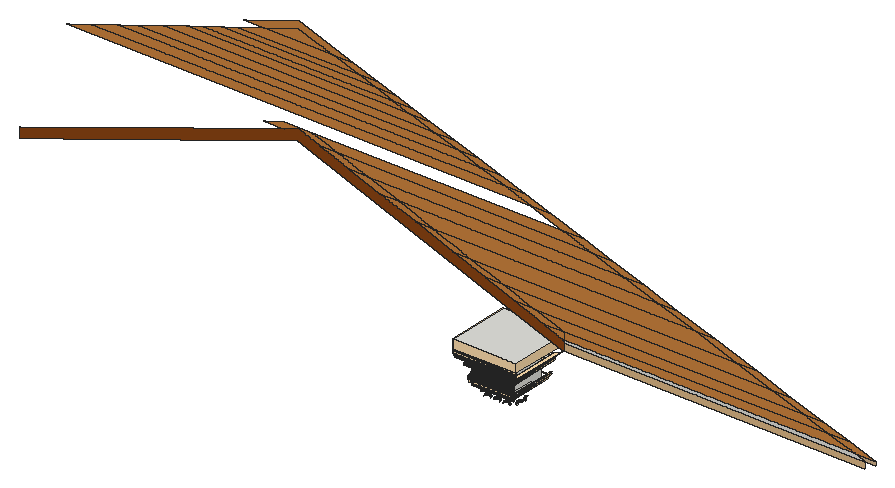
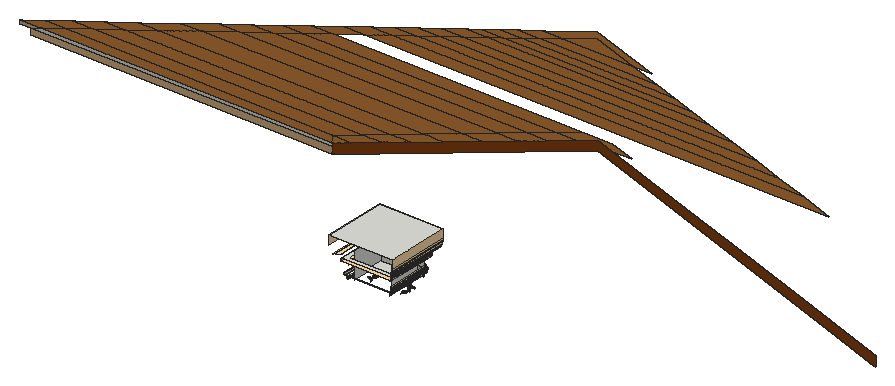
# SketchUp Ruby script. Lengths in inches.
U = 1.inch
M = Sketchup.active_model
def pt(a) = Geom::Point3d.new(a.map { |v| v * U })
def face(e, loops, mat)
  f = e.add_face(loops[0].map { |a| pt(a) })
  loops[1..].each { |l| e.add_face(l.map { |a| pt(a) }).erase! }
  f.material = f.back_material = mat if mat
  f
end
# faces: each face lists its corners as indices into pts; further lists are holes
def faces(e, pts, list, mat = nil) = list.each { |f| face(e, (f[0].is_a?(Array) ? f : [f]).map { |l| l.map { |i| pts[i] } }, mat) }
# xy, xz, yz: faces in a plane at the given z, y or x. An outline is a flat list of corners, or four numbers for a rectangle; further outlines are holes
def ring(l) = l.size == 4 ? [[l[0], l[1]], [l[2], l[1]], [l[2], l[3]], [l[0], l[3]]] : l.each_slice(2).to_a
def flat(e, list, mat, &to3) = list.each { |f| face(e, (f[0].is_a?(Array) ? f : [f]).map { |l| ring(l).map { |u, v| to3.(u, v) } }, mat) }
def xy(e, z, list, mat = nil) = flat(e, list, mat) { |x, y| [x, y, z] }
def xz(e, y, list, mat = nil) = flat(e, list, mat) { |x, z| [x, y, z] }
def yz(e, x, list, mat = nil) = flat(e, list, mat) { |y, z| [x, y, z] }
def lines(e, pts, list) = list.each { |a, b| e.add_line(pt(pts[a]), pt(pts[b])) }
# prism: a flat outline (further loops are holes) pulled along v
def prism(e, loops, v, mat = nil)
  f = face(e, loops, mat); d = Geom::Vector3d.new(v.map { |x| x * U })
  f.pushpull(f.normal.samedirection?(d) ? d.length : -d.length)
end
def box(e, o, s, mat = nil) = prism(e, [[o, [o[0] + s[0], o[1], o[2]], [o[0] + s[0], o[1] + s[1], o[2]], [o[0], o[1] + s[1], o[2]]]], [0, 0, s[2]], mat)
def at(x, y, z, deg = 0) = Geom::Transformation.translation(pt([x, y, z])) * Geom::Transformation.rotation(ORIGIN, Z_AXIS, deg.degrees)
def axes(o, x, y, z) = Geom::Transformation.new([*x, 0, *y, 0, *z, 0, *pt(o).to_a, 1])
def part(name) = M.definitions.add(name)
# library, detail: a bought-in or finely detailed component or shape, given as its bounding box
def library(name, o, s) = part(name).tap { |d| box(d.entities, o, s) }
def detail(e, o, s) = box(e.add_group.entities, o, s)
def put(e, d, t, mat = nil) = e.add_instance(d, t).tap { |i| i.material = mat if mat }
def group(e, t, mat = nil) = e.add_group.tap { |g| g.transformation = t; g.material = mat if mat }.entities
root = M.entities
M.materials.add("[0033_NavajoWhite]").color = [255, 222, 173]
M.materials.add("[0035_Tan]").color = [210, 180, 140]
M.materials.add("[0036_BurlyWood]").color = [222, 184, 135]
M.materials.add("[0040_Peru]").color = [205, 133, 63]
M.materials.add("[0043_SaddleBrown]").color = [139, 69, 19]
xy(root,95.99,[[231.46,8.1,244.45,14.59]])
xy(root,96.66,[[[230.87,7.51,245.04,21.68],[230.94,7.58,244.97,21.61]]],"[0033_NavajoWhite]")
xy(root,100.56,[[[230.28,6.92,245.64,22.27],[231.46,8.1,244.45,21.09]]],"[0033_NavajoWhite]")
xy(root,101.46,[[[230.28,6.92,245.64,22.27],[231.46,8.1,244.45,21.09]]])
xy(root,102.72,[[230.08,6.72,230.28,6.92,245.64,6.92,245.83,6.72]])
xy(root,102.72,[[229.3,5.93,229.3,23.25,230.28,22.27,230.28,6.92,230.08,6.72],[229.3,5.93,230.08,6.72,245.83,6.72,246.62,5.93],[246.62,5.93,245.83,6.72,245.64,6.92,245.64,22.27,245.83,22.47,246.62,23.25]],"[0033_NavajoWhite]")
xy(root,102.86,[[232.25,9.67,243.67,14.59]])
xy(root,105.42,[[230.08,6.72,245.83,14.59]])
xy(root,108.125,[[228.12,4.75,247.8,24.44]])
xz(root,4.75,[[262.6,116.78,262.6,117,261.99,117,262.52,116.81],[262.6,119,356.68,119,353.68,120,262.6,120],[262.6,119.97,262.6,120,262.52,120]])
xz(root,4.75,[[228.12,105.42,247.8,108.125]],"[0033_NavajoWhite]")
xz(root,4.75,[[356.68,119,360,119,360,120,353.68,120]],"[0035_Tan]")
xz(root,4.75,[[262.6,117,356.68,119]],"[0036_BurlyWood]")
xz(root,4.75,[[262.52,120,262.6,120,262.6,122.1,256.71,122.1],[262.6,120,353.68,120,345.49,122.73,262.6,122.1],[353.68,120,360,120,351.8125,122.73,345.49,122.73],[256.71,122.1,262.6,122.1,253.29,125.46,247.4,125.46],[262.6,122.1,345.49,122.73,337.3,125.46,253.29,125.46],
  [345.49,122.73,351.8125,122.73,343.625,125.46,337.3,125.46],[247.4,125.46,253.29,125.46,243.99,128.82,238.1,128.82],[253.29,125.46,337.3,125.46,327.22,128.82,243.99,128.82],[337.3,125.46,343.625,125.46,333.54,128.82,327.22,128.82],[238.1,128.82,243.99,128.82,234.04,132.41,228.15,132.41],
  [243.99,128.82,327.22,128.82,316.44,132.41,234.04,132.41],[327.22,128.82,333.54,128.82,322.77,132.41,316.44,132.41],[228.15,132.41,234.04,132.41,222.03,136.75,216.15,136.75],[234.04,132.41,316.44,132.41,303.43,136.75,222.03,136.75],[316.44,132.41,322.77,132.41,309.76,136.75,303.43,136.75],
  [216.15,136.75,222.03,136.75,211.26,140.64,205.37,140.64],[222.03,136.75,303.43,136.75,291.76,140.64,211.26,140.64],[303.43,136.75,309.76,136.75,298.08,140.64,291.76,140.64],[205.37,140.64,211.26,140.64,201.59,144.13,195.7,144.13],[211.26,140.64,291.76,140.64,281.28,144.13,201.59,144.13],
  [291.76,140.64,298.08,140.64,287.61,144.13,281.28,144.13],[195.7,144.13,201.59,144.13,192.4375,147.4375,186.55,147.4375],[201.59,144.13,281.28,144.13,271.37,147.4375,192.4375,147.4375],[281.28,144.13,287.61,144.13,277.69,147.4375,271.37,147.4375],[186.55,147.4375,192.4375,147.4375,184.29,150.38,175.49,150.38,169.17,148.21,175.27,148.21,179.96,149.82,180,149.8],
  [192.4375,147.4375,271.37,147.4375,262.54,150.38,184.29,150.38],[271.37,147.4375,277.69,147.4375,268.86,150.38,262.54,150.38],[262.54,150.38,268.86,150.38,258.67,153.78,252.34,153.78],[107.66,153.78,252.34,153.78,244.33,156.45,115.67,156.45],[252.34,153.78,258.67,153.78,250.66,156.45,244.33,156.45],
  [115.67,156.45,244.33,156.45,236.39,159.09,123.61,159.09],[244.33,156.45,250.66,156.45,242.72,159.09,236.39,159.09],[123.61,159.09,236.39,159.09,229.64,161.35,130.36,161.35],[236.39,159.09,242.72,159.09,235.96,161.35,229.64,161.35],[130.36,161.35,229.64,161.35,222.01,163.89,137.99,163.89],
  [229.64,161.35,235.96,161.35,228.33,163.89,222.01,163.89],[137.99,163.89,222.01,163.89,214.75,166.31,145.25,166.31],[222.01,163.89,228.33,163.89,221.07,166.31,214.75,166.31],[145.25,166.31,214.75,166.31,209.51,168.05,150.49,168.05],[214.75,166.31,221.07,166.31,215.69,168.1,209.51,168.05],
  [150.49,168.05,209.51,168.05,203.74,169.98,156.26,169.98],[209.51,168.05,215.69,168.1,209.93,170.02,203.74,169.98],[156.26,169.98,203.74,169.98,198.59,171.69,161.41,171.69],[203.74,169.98,209.93,170.02,204.77,171.74,198.59,171.69],[161.41,171.69,198.59,171.69,190.82,174.29,169.18,174.29],
  [198.59,171.69,204.77,171.74,197,174.33,190.82,174.29],[162.86,174.29,169.18,174.29,180,177.89,190.82,174.29,197,174.33,180,180],[169.18,174.29,190.82,174.29,180,177.89]],"[0040_Peru]")
xz(root,4.75,[[93.16,117,93.71,117,106.86,121.52,179.96,146.625,247.8,122.125,261.99,117,262.6,117,262.6,119.97,262.52,120,256.71,122.1,247.4,125.46,238.1,128.82,228.15,132.41,216.15,136.75,205.37,140.64,195.7,144.13,186.55,147.4375,180,149.8,164.92,144.62,147.21,138.54,139.33,135.83,120.1,129.23,93.21,120,93.16,119.98]],"[0043_SaddleBrown]")
xz(root,6.72,[[230.08,102.72,245.83,105.42]])
xz(root,7.11,[[230.47,101.95,245.44,101.95,245.4375,102.09,230.48,102.09],[230.48,102.09,245.4375,102.09,245.44,102.23,230.47,102.23]],"[0033_NavajoWhite]")
xz(root,7.58,[[230.94,95.99,244.97,96.66]],"[0033_NavajoWhite]")
xz(root,8.1,[[231.46,94.95,244.45,95.1],[231.46,95.1,244.45,95.99],[231.46,95.99,244.45,97.5625],[231.46,97.5625,244.45,99.87],[231.46,99.87,244.45,100.56],
  [231.46,100.56,244.45,101.46]])
xz(root,9.67,[[232.25,94.95,243.67,102.86]])
yz(root,228.12,[[4.75,105.42,24.44,108.125]],"[0033_NavajoWhite]")
yz(root,231.46,[[8.1,95.99,14.59,97.5625]])
yz(root,232.25,[[9.67,94.95,19.51,102.86]])
yz(root,243.67,[[9.67,94.95,19.51,102.86]])
yz(root,244.45,[[8.1,95.99,14.59,97.5625]])
yz(root,247.8,[[4.75,105.42,24.44,108.125]],"[0033_NavajoWhite]")
p = [[234.09,9.92,92.48],[234.05,9.67,92.48],[234.02,9.67,92.25],[234.05,9.93,92.25],[235.96,9.93,92.25],[235.99,9.67,92.25],
  [235.96,9.67,92.48],[235.92,9.92,92.48],[237.04,9.92,92.48],[237.01,9.67,92.48],[236.97,9.67,92.25],[237.01,9.93,92.25],
  [238.91,9.93,92.25],[238.94,9.67,92.25],[238.91,9.67,92.48],[238.875,9.92,92.48],[239.99,9.92,92.48],[239.96,9.67,92.48],
  [239.93,9.67,92.25],[239.96,9.93,92.25],[241.86,9.93,92.25],[241.9,9.67,92.25],[241.86,9.67,92.48],[241.83,9.92,92.48],
  [234.15,10.16,92.25],[234.18,10.15,92.48],[235.83,10.15,92.48],[235.86,10.16,92.25],[237.11,10.16,92.25],[237.14,10.15,92.48],
  [238.78,10.15,92.48],[238.8125,10.16,92.25],[240.06,10.16,92.25],[240.09,10.15,92.48],[241.73,10.15,92.48],[241.76,10.16,92.25],
  [234.31,10.37,92.25],[234.33,10.34,92.48],[235.68,10.34,92.48],[235.7,10.37,92.25],[237.26,10.37,92.25],[237.29,10.34,92.48],
  [238.63,10.34,92.48],[238.65,10.37,92.25],[240.22,10.37,92.25],[240.24,10.34,92.48],[241.58,10.34,92.48],[241.61,10.37,92.25],
  [234.51,10.52,92.25],[234.53,10.49,92.48],[235.48,10.49,92.48],[235.5,10.52,92.25],[237.47,10.52,92.25],[237.48,10.49,92.48],
  [238.43,10.49,92.48],[238.45,10.52,92.25],[240.42,10.52,92.25],[240.4375,10.49,92.48],[241.39,10.49,92.48],[241.4,10.52,92.25],
  [234.75,10.62,92.25],[234.76,10.59,92.48],[235.25,10.59,92.48],[235.26,10.62,92.25],[237.7,10.62,92.25],[237.71,10.59,92.48],
  [238.2,10.59,92.48],[238.21,10.62,92.25],[240.66,10.62,92.25],[240.67,10.59,92.48],[241.16,10.59,92.48],[241.17,10.62,92.25],
  [235.01,10.66,92.25],[235.01,10.62,92.48],[237.96,10.66,92.25],[237.96,10.62,92.48],[240.91,10.66,92.25],[240.91,10.62,92.48],
  [234.18,9.89,92.7],[234.15,9.67,92.7],[235.86,9.67,92.7],[235.83,9.89,92.7],[237.14,9.89,92.7],[237.11,9.67,92.7],
  [238.8125,9.67,92.7],[238.78,9.89,92.7],[240.09,9.89,92.7],[240.06,9.67,92.7],[241.76,9.67,92.7],[241.73,9.89,92.7],
  [234.27,10.1,92.7],[235.74,10.1,92.7],[237.22,10.1,92.7],[238.7,10.1,92.7],[240.17,10.1,92.7],[241.65,10.1,92.7],
  [234.4,10.27,92.7],[235.61,10.27,92.7],[237.36,10.27,92.7],[238.5625,10.27,92.7],[240.31,10.27,92.7],[241.51,10.27,92.7],
  [234.58,10.41,92.7],[235.43,10.41,92.7],[237.53,10.41,92.7],[238.38,10.41,92.7],[240.48,10.41,92.7],[241.34,10.41,92.7],
  [234.78,10.49,92.7],[235.23,10.49,92.7],[237.74,10.49,92.7],[238.18,10.49,92.7],[240.69,10.49,92.7],[241.13,10.49,92.7],
  [235.01,10.52,92.7],[237.96,10.52,92.7],[240.91,10.52,92.7],[232.5,10.6875,92.51],[232.25,10.66,92.51],[232.25,10.6875,92.74],
  [232.5,10.72,92.74],[232.73,10.82,92.74],[232.74,10.79,92.51],[243.17,10.79,92.51],[243.19,10.82,92.74],[243.42,10.72,92.74],
  [243.41,10.6875,92.51],[243.67,10.66,92.51],[243.67,10.6875,92.74],[232.92,10.97,92.74],[232.95,10.94,92.51],[242.97,10.94,92.51],
  [242.99,10.97,92.74],[233.07,11.16,92.74],[233.1,11.15,92.51],[242.81,11.15,92.51],[242.84,11.16,92.74],[233.17,11.39,92.74],
  [233.2,11.39,92.51],[242.72,11.39,92.51],[242.75,11.39,92.74],[233.2,11.64,92.74],[233.23,11.64,92.51],[242.68,11.64,92.51],
  [242.72,11.64,92.74],[233.17,11.89,92.74],[233.2,11.89,92.51],[242.72,11.89,92.51],[242.75,11.89,92.74],[233.07,12.12,92.74],
  [233.1,12.13,92.51],[242.81,12.13,92.51],[242.84,12.12,92.74],[232.92,12.3125,92.74],[232.95,12.34,92.51],[242.97,12.34,92.51],
  [242.99,12.3125,92.74],[232.73,12.46,92.74],[232.74,12.49,92.51],[243.17,12.49,92.51],[243.19,12.46,92.74],[232.5,12.56,92.74],
  [232.5,12.59,92.51],[243.41,12.59,92.51],[243.42,12.56,92.74],[232.25,12.59,92.74],[232.25,12.625,92.51],[243.67,12.59,92.74],
  [243.67,12.625,92.51],[232.5,13.64,92.51],[232.25,13.61,92.51],[232.25,13.64,92.74],[232.5,13.67,92.74],[232.73,13.77,92.74],
  [232.74,13.74,92.51],[243.17,13.74,92.51],[243.19,13.77,92.74],[243.42,13.67,92.74],[243.41,13.64,92.51],[243.67,13.61,92.51],
  [243.67,13.64,92.74],[232.92,13.92,92.74],[232.95,13.9,92.51],[242.97,13.9,92.51],[242.99,13.92,92.74],[233.07,14.12,92.74],
  [233.1,14.1,92.51],[242.81,14.1,92.51],[242.84,14.12,92.74],[233.17,14.35,92.74],[233.2,14.34,92.51],[242.72,14.34,92.51],
  [242.75,14.35,92.74],[233.2,14.59,92.74],[233.23,14.59,92.51],[242.68,14.59,92.51],[242.72,14.59,92.74],[234.33,9.85,92.89],
  [234.31,9.67,92.89],[235.7,9.67,92.89],[235.68,9.85,92.89],[237.29,9.85,92.89],[237.26,9.67,92.89],[238.65,9.67,92.89],
  [238.63,9.85,92.89],[240.24,9.85,92.89],[240.22,9.67,92.89],[241.61,9.67,92.89],[241.58,9.85,92.89],[234.4,10.02,92.89],
  [235.61,10.02,92.89],[237.36,10.02,92.89],[238.5625,10.02,92.89],[240.31,10.02,92.89],[241.51,10.02,92.89],[234.51,10.16,92.89],
  [235.5,10.16,92.89],[237.47,10.16,92.89],[238.45,10.16,92.89],[240.42,10.16,92.89],[241.4,10.16,92.89],[234.66,10.27,92.89],
  [235.35,10.27,92.89],[237.61,10.27,92.89],[238.31,10.27,92.89],[240.5625,10.27,92.89],[241.26,10.27,92.89],[234.83,10.34,92.89],
  [235.01,10.37,92.89],[235.1875,10.34,92.89],[237.78,10.34,92.89],[237.96,10.37,92.89],[238.14,10.34,92.89],[240.73,10.34,92.89],
  [240.91,10.37,92.89],[241.09,10.34,92.89],[232.25,10.79,92.96],[232.47,10.82,92.96],[232.68,10.9,92.96],[243.24,10.9,92.96],
  [243.45,10.82,92.96],[243.67,10.79,92.96],[232.85,11.04,92.96],[243.0625,11.04,92.96],[232.99,11.21,92.96],[242.93,11.21,92.96],
  [233.07,11.42,92.96],[242.84,11.42,92.96],[233.1,11.64,92.96],[242.81,11.64,92.96],[233.07,11.86,92.96],[242.84,11.86,92.96],
  [232.99,12.07,92.96],[242.93,12.07,92.96],[232.85,12.24,92.96],[243.0625,12.24,92.96],[232.68,12.38,92.96],[243.24,12.38,92.96],
  [232.47,12.46,92.96],[243.45,12.46,92.96],[232.25,12.49,92.96],[243.67,12.49,92.96],[232.25,13.74,92.96],[232.47,13.77,92.96],
  [243.45,13.77,92.96],[243.67,13.74,92.96],[232.68,13.85,92.96],[243.24,13.85,92.96],[232.85,13.99,92.96],[243.0625,13.99,92.96],
  [232.99,14.17,92.96],[242.93,14.17,92.96],[233.07,14.37,92.96],[242.84,14.37,92.96],[233.1,14.59,92.96],[242.81,14.59,92.96],
  [234.53,9.8,93.03],[234.51,9.67,93.03],[235.5,9.67,93.03],[235.48,9.8,93.03],[237.48,9.8,93.03],[237.47,9.67,93.03],
  [238.45,9.67,93.03],[238.43,9.8,93.03],[240.4375,9.8,93.03],[240.42,9.67,93.03],[241.4,9.67,93.03],[241.39,9.8,93.03],
  [234.58,9.92,93.03],[235.43,9.92,93.03],[237.53,9.92,93.03],[238.38,9.92,93.03],[240.48,9.92,93.03],[241.34,9.92,93.03],
  [234.66,10.02,93.03],[235.35,10.02,93.03],[237.61,10.02,93.03],[238.31,10.02,93.03],[240.5625,10.02,93.03],[241.26,10.02,93.03],
  [234.76,10.1,93.03],[235.25,10.1,93.03],[237.71,10.1,93.03],[238.2,10.1,93.03],[240.67,10.1,93.03],[241.16,10.1,93.03],
  [234.88,10.15,93.03],[235.01,10.16,93.03],[235.13,10.15,93.03],[237.83,10.15,93.03],[237.96,10.16,93.03],[238.09,10.15,93.03],
  [240.78,10.15,93.03],[240.91,10.16,93.03],[241.04,10.15,93.03],[234.76,9.74,93.12],[234.75,9.67,93.12],[234.78,9.8,93.12],
  [235.23,9.8,93.12],[235.25,9.74,93.12],[235.26,9.67,93.12],[237.71,9.74,93.12],[237.7,9.67,93.12],[237.74,9.8,93.12],
  [238.21,9.67,93.12],[238.2,9.74,93.12],[238.18,9.8,93.12],[240.67,9.74,93.12],[240.66,9.67,93.12],[240.69,9.8,93.12],
  [241.13,9.8,93.12],[241.16,9.74,93.12],[241.17,9.67,93.12],[234.83,9.85,93.12],[235.1875,9.85,93.12],[237.78,9.85,93.12],
  [238.14,9.85,93.12],[240.73,9.85,93.12],[241.09,9.85,93.12],[234.88,9.89,93.12],[234.94,9.92,93.12],[235.01,9.93,93.12],
  [235.07,9.92,93.12],[235.13,9.89,93.12],[237.83,9.89,93.12],[237.89,9.92,93.12],[237.96,9.93,93.12],[238.02,9.92,93.12],
  [238.09,9.89,93.12],[240.78,9.89,93.12],[240.85,9.92,93.12],[240.91,9.93,93.12],[240.98,9.92,93.12],[241.04,9.89,93.12],
  [232.25,10.94,93.15],[232.43,10.97,93.15],[232.6,11.04,93.15],[243.32,11.04,93.15],[243.49,10.97,93.15],[243.67,10.94,93.15],
  [232.74,11.15,93.15],[243.17,11.15,93.15],[232.85,11.29,93.15],[243.0625,11.29,93.15],[232.92,11.46,93.15],[242.99,11.46,93.15],
  [232.95,11.64,93.15],[242.97,11.64,93.15],[232.92,11.82,93.15],[242.99,11.82,93.15],[232.85,11.99,93.15],[243.0625,11.99,93.15],
  [232.74,12.13,93.15],[243.17,12.13,93.15],[232.6,12.24,93.15],[243.32,12.24,93.15],[232.43,12.3125,93.15],[243.49,12.3125,93.15],
  [232.25,12.34,93.15],[243.67,12.34,93.15],[232.25,13.9,93.15],[232.43,13.92,93.15],[243.49,13.92,93.15],[243.67,13.9,93.15],
  [232.6,13.99,93.15],[243.32,13.99,93.15],[232.74,14.1,93.15],[243.17,14.1,93.15],[232.85,14.24,93.15],[243.0625,14.24,93.15],
  [232.92,14.41,93.15],[242.99,14.41,93.15],[232.95,14.59,93.15],[242.97,14.59,93.15],[235.01,9.67,93.15],[237.96,9.67,93.15],
  [240.91,9.67,93.15],[232.25,11.15,93.29],[232.38,11.16,93.29],[243.54,11.16,93.29],[243.67,11.15,93.29],[232.5,11.21,93.29],
  [232.6,11.29,93.29],[243.32,11.29,93.29],[243.42,11.21,93.29],[232.68,11.39,93.29],[243.24,11.39,93.29],[232.73,11.51,93.29],
  [243.19,11.51,93.29],[232.74,11.64,93.29],[243.17,11.64,93.29],[232.73,11.77,93.29],[243.19,11.77,93.29],[232.68,11.89,93.29],
  [243.24,11.89,93.29],[232.6,11.99,93.29],[243.32,11.99,93.29],[232.5,12.07,93.29],[243.42,12.07,93.29],[232.38,12.12,93.29],
  [232.25,12.13,93.29],[243.54,12.12,93.29],[243.67,12.13,93.29],[232.25,14.1,93.29],[232.38,14.12,93.29],[232.5,14.17,93.29],
  [243.42,14.17,93.29],[243.54,14.12,93.29],[243.67,14.1,93.29],[232.6,14.24,93.29],[243.32,14.24,93.29],[232.68,14.35,93.29],
  [243.24,14.35,93.29],[232.73,14.47,93.29],[243.19,14.47,93.29],[232.74,14.59,93.29],[243.17,14.59,93.29],[232.25,11.39,93.38],
  [232.32,11.39,93.38],[243.6,11.39,93.38],[243.67,11.39,93.38],[232.38,11.42,93.38],[232.43,11.46,93.38],[243.49,11.46,93.38],
  [243.54,11.42,93.38],[232.47,11.51,93.38],[243.45,11.51,93.38],[232.5,11.57,93.38],[243.42,11.57,93.38],[232.5,11.64,93.38],
  [243.41,11.64,93.38],[232.5,11.71,93.38],[243.42,11.71,93.38],[232.47,11.77,93.38],[243.45,11.77,93.38],[232.43,11.82,93.38],
  [232.38,11.86,93.38],[243.49,11.82,93.38],[243.54,11.86,93.38],[232.32,11.89,93.38],[232.25,11.89,93.38],[243.6,11.89,93.38],
  [243.67,11.89,93.38],[232.25,14.34,93.38],[232.32,14.35,93.38],[232.38,14.37,93.38],[243.54,14.37,93.38],[243.6,14.35,93.38],
  [243.67,14.34,93.38],[232.43,14.41,93.38],[232.47,14.47,93.38],[243.45,14.47,93.38],[243.49,14.41,93.38],[232.5,14.53,93.38],
  [243.42,14.53,93.38],[232.5,14.59,93.38],[243.41,14.59,93.38],[232.25,11.64,93.41],[243.67,11.64,93.41],[232.25,14.59,93.41],
  [243.67,14.59,93.41],[231.45,8.09,95.25],[231.46,8.1,95.1],[244.45,8.1,95.1],[244.47,8.09,95.25],[231.43,8.06,95.4],
  [244.49,8.06,95.4],[231.4,8.03,95.53],[244.52,8.03,95.53],[231.4,21.15,95.53],[231.43,21.12,95.4],[244.49,21.12,95.4],
  [244.52,21.15,95.53],[231.36,8,95.66],[244.55,8,95.66],[231.36,21.1875,95.66],[244.55,21.1875,95.66],[231.32,7.95,95.77],
  [244.6,7.95,95.77],[231.32,21.24,95.77],[244.6,21.24,95.77],[231.26,7.9,95.86],[244.65,7.9,95.86],[231.14,7.78,95.98],
  [231.2,7.84,95.93],[244.71,7.84,95.93],[244.78,7.78,95.98],[231.14,21.41,95.98],[231.2,21.35,95.93],[244.71,21.35,95.93],
  [244.78,21.41,95.98],[231.11,7.74,95.99],[244.81,7.74,95.99],[230.73,7.37,96.79],[230.77,7.41,96.72],[245.14,7.41,96.72],
  [245.18,7.37,96.79],[230.73,21.82,96.79],[230.77,21.78,96.72],[230.82,7.45,96.68],[245.1,7.45,96.68],[230.82,21.73,96.68],
  [245.14,21.78,96.72],[245.18,21.82,96.79],[230.87,7.51,96.66],[245.04,7.51,96.66],[230.87,21.68,96.66],[230.7,7.34,96.89],
  [245.22,7.34,96.89],[230.7,21.85,96.89],[245.22,21.85,96.89],[230.68,7.32,96.99],[245.24,7.32,96.99],[230.68,21.87,96.99],
  [230.67,7.31,97.11],[245.24,7.31,97.11],[230.67,21.875,97.11],[230.68,7.32,97.23],[245.24,7.32,97.23],[230.68,21.87,97.23],
  [230.7,7.34,97.34],[245.22,7.34,97.34],[230.7,21.85,97.34],[230.73,7.37,97.43],[245.18,7.37,97.43],[230.73,21.82,97.43],
  [245.22,21.85,97.34],[245.18,21.82,97.43],[230.77,7.41,97.5],[245.14,7.41,97.5],[230.77,21.78,97.5],[245.14,21.78,97.5],
  [230.82,7.45,97.55],[245.1,7.45,97.55],[230.82,21.73,97.55],[230.87,7.51,97.5625],[245.04,7.51,97.5625],[230.87,21.68,97.5625],
  [230.97,7.61,97.74],[244.95,7.61,97.74],[230.97,21.58,97.74],[231.0625,7.7,97.93],[244.85,7.7,97.93],[231.15,7.78,98.14],
  [244.77,7.78,98.14],[231.15,21.4,98.14],[231.0625,21.49,97.93],[231.22,7.86,98.375],[244.69,7.86,98.375],[231.29,7.92,98.62],
  [244.625,7.92,98.62],[231.35,7.98,98.875],[244.57,7.98,98.875],[231.39,8.03,99.14],[244.52,8.03,99.14],[231.43,8.0625,99.42],
  [244.49,8.0625,99.42],[231.45,8.09,99.7],[244.46,8.09,99.7],[231.45,21.1,99.7],[231.43,21.12,99.42],[244.49,21.12,99.42],
  [244.46,21.1,99.7],[231.46,8.1,99.87],[244.45,8.1,99.87],[230.14,6.78,100.6875],[230.18,6.82,100.62],[245.73,6.82,100.62],
  [245.77,6.78,100.6875],[230.23,6.86,100.57],[245.6875,6.86,100.57],[230.28,6.92,100.56],[245.64,6.92,100.56],[230.23,22.32,100.57],
  [230.28,22.27,100.56],[230.11,6.74,100.78],[245.81,6.74,100.78],[230.11,22.44,100.78],[230.14,22.41,100.6875],[230.09,6.73,100.89],
  [245.83,6.73,100.89],[230.09,22.46,100.89],[245.81,22.44,100.78],[245.83,22.46,100.89],[230.08,6.72,101.01],[245.83,6.72,101.01],
  [230.08,22.47,101.01],[230.09,6.73,101.125],[245.83,6.73,101.125],[230.09,22.46,101.125],[230.11,6.74,101.23],[245.81,6.74,101.23],
  [230.11,22.44,101.23],[245.83,22.46,101.125],[245.81,22.44,101.23],[230.14,6.78,101.33],[245.77,6.78,101.33],[230.14,22.41,101.33],
  [230.18,6.82,101.4],[245.73,6.82,101.4],[230.23,6.86,101.44],[245.6875,6.86,101.44],[230.28,6.92,101.46],[245.64,6.92,101.46],
  [230.28,22.27,101.46],[230.23,22.32,101.44],[245.58,6.97,101.52],[230.34,6.97,101.52],[230.34,22.22,101.52],[245.58,22.22,101.52],
  [245.64,22.27,101.46],[245.53,7.02,101.6],[230.38,7.02,101.6],[230.38,22.17,101.6],[245.49,7.06,101.7],[230.42,7.06,101.7],
  [230.42,22.13,101.7],[245.46,7.09,101.82],[230.45,7.09,101.82],[230.45,22.1,101.82],[245.44,7.11,101.95],[230.47,7.11,101.95],
  [245.44,7.11,102.23],[245.46,7.09,102.36],[230.45,7.09,102.36],[230.47,7.11,102.23],[245.49,7.06,102.48],[230.42,7.06,102.48],
  [230.45,22.1,102.36],[230.42,22.13,102.48],[245.53,7.02,102.58],[230.38,7.02,102.58],[230.38,22.17,102.58],[245.58,6.97,102.66],
  [230.34,6.97,102.66],[230.34,22.22,102.66],[246.94,5.61,102.73],[247.1,5.45,102.82],[228.82,5.45,102.82],[228.98,5.61,102.73],
  [228.82,23.73,102.82],[228.98,23.58,102.73],[246.94,23.58,102.73],[247.1,23.73,102.82],[246.78,5.77,102.7],[229.14,5.77,102.7],
  [229.14,23.41,102.7],[246.62,5.93,102.72],[229.3,5.93,102.72],[229.3,23.25,102.72],[245.64,6.92,102.72],[230.28,6.92,102.72],
  [230.28,22.27,102.72],[245.64,22.27,102.72],[245.58,22.22,102.66],[247.25,5.3,102.96],[228.67,5.3,102.96],[228.67,23.88,102.96],
  [247.38,5.17,103.15],[228.53,5.17,103.15],[247.51,5.05,103.39],[228.41,5.05,103.39],[228.41,24.14,103.39],[228.53,24.02,103.15],
  [247.61,4.94,103.68],[228.31,4.94,103.68],[228.31,24.24,103.68],[247.7,4.86,103.99],[228.22,4.86,103.99],[247.76,4.79,104.33],
  [228.16,4.79,104.33],[228.16,24.39,104.33],[228.22,24.33,103.99],[247.8,4.75,104.6875],[228.12,4.75,104.6875],[228.12,24.43,104.6875],
  [247.8125,4.74,105.05],[228.11,4.74,105.05],[247.8,4.75,105.42],[228.12,4.75,105.42],[228.12,24.44,105.42],[228.11,24.45,105.05]]
faces(root,p,[[0,1,2,3],[4,5,6,7],[8,9,10,11],[12,13,14,15],[16,17,18,19],[20,21,22,23],[0,3,24,25],[26,27,4,7],
  [8,11,28,29],[30,31,12,15],[16,19,32,33],[34,35,20,23],[25,24,36,37],[38,39,27,26],[29,28,40,41],[42,43,31,30],
  [33,32,44,45],[46,47,35,34],[37,36,48,49],[50,51,39,38],[41,40,52,53],[54,55,43,42],[45,44,56,57],[58,59,47,46],
  [49,48,60,61],[62,63,51,50],[53,52,64,65],[66,67,55,54],[57,56,68,69],[70,71,59,58],[61,60,72,73],[73,72,63,62],
  [65,64,74,75],[75,74,67,66],[69,68,76,77],[77,76,71,70],[78,79,1,0],[7,6,80,81],[82,83,9,8],[15,14,84,85],
  [86,87,17,16],[23,22,88,89],[78,0,25,90],[91,26,7,81],[82,8,29,92],[93,30,15,85],[86,16,33,94],[95,34,23,89],
  [90,25,37,96],[97,38,26,91],[92,29,41,98],[99,42,30,93],[94,33,45,100],[101,46,34,95],[96,37,49,102],[103,50,38,97],
  [98,41,53,104],[105,54,42,99],[100,45,57,106],[107,58,46,101],[102,49,61,108],[109,62,50,103],[104,53,65,110],[111,66,54,105],
  [106,57,69,112],[113,70,58,107],[108,61,73,114],[114,73,62,109],[110,65,75,115],[115,75,66,111],[112,69,77,116],[116,77,70,113],
  [197,198,79,78],[81,80,199,200],[201,202,83,82],[85,84,203,204],[205,206,87,86],[89,88,207,208],[197,78,90,209],[210,91,81,200],
  [201,82,92,211],[212,93,85,204],[205,86,94,213],[214,95,89,208],[209,90,96,215],[216,97,91,210],[211,92,98,217],[218,99,93,212],
  [213,94,100,219],[220,101,95,214],[215,96,102,221],[222,103,97,216],[217,98,104,223],[224,105,99,218],[219,100,106,225],[226,107,101,220],
  [221,102,108,227],[227,108,114,228],[228,114,109,229],[229,109,103,222],[223,104,110,230],[230,110,115,231],[231,115,111,232],[232,111,105,224],
  [225,106,112,233],[233,112,116,234],[234,116,113,235],[235,113,107,226],[276,277,198,197],[200,199,278,279],[280,281,202,201],[204,203,282,283],
  [284,285,206,205],[208,207,286,287],[276,197,209,288],[289,210,200,279],[280,201,211,290],[291,212,204,283],[284,205,213,292],[293,214,208,287],
  [288,209,215,294],[295,216,210,289],[290,211,217,296],[297,218,212,291],[292,213,219,298],[299,220,214,293],[294,215,221,300],[301,222,216,295],
  [296,217,223,302],[303,224,218,297],[298,219,225,304],[305,226,220,299],[300,221,227,306],[306,227,228,307],[307,228,229,308],[308,229,222,301],
  [302,223,230,309],[309,230,231,310],[310,231,232,311],[311,232,224,303],[304,225,233,312],[312,233,234,313],[313,234,235,314],[314,235,226,305],
  [315,316,277,276],[315,276,288,317],[318,289,279,319],[279,278,320,319],[321,322,281,280],[321,280,290,323],[283,282,324,325],[326,291,283,325],
  [327,328,285,284],[327,284,292,329],[330,293,287,331],[287,286,332,331],[317,288,294,333],[334,295,289,318],[323,290,296,335],[336,297,291,326],
  [329,292,298,337],[338,299,293,330],[333,294,300,339],[339,300,306,340],[340,306,307,341],[341,307,308,342],[343,301,295,334],[342,308,301,343],
  [335,296,302,344],[344,302,309,345],[345,309,310,346],[347,311,303,348],[346,310,311,347],[348,303,297,336],[337,298,304,349],[349,304,312,350],
  [350,312,313,351],[351,313,314,352],[353,305,299,338],[352,314,305,353],[315,394,316],[394,315,317],[394,317,333],[394,333,339],
  [394,339,340],[394,340,341],[319,320,394],[394,318,319],[394,334,318],[394,343,334],[394,342,343],[394,341,342],
  [321,395,322],[395,321,323],[395,323,335],[395,335,344],[395,344,345],[395,345,346],[325,324,395],[395,326,325],
  [395,336,326],[395,348,336],[395,347,348],[395,346,347],[327,396,328],[396,327,329],[396,329,337],[396,337,349],
  [396,349,350],[396,350,351],[331,332,396],[396,330,331],[396,338,330],[396,353,338],[396,352,353],[396,351,352],
  [481,482,483,484],[485,481,484,486],[487,485,486,488],[487,489,490,485],[486,491,492,488],[493,487,488,494],[493,495,489,487],[488,492,496,494],
  [497,493,494,498],[497,499,495,493],[494,496,500,498],[501,497,498,502],[503,504,505,506],[503,507,508,504],[504,501,502,505],[505,509,510,506],
  [511,503,506,512],[513,514,515,516],[513,517,518,514],[514,519,520,515],[514,518,521,519],[515,522,523,516],[519,524,525,520],[519,521,526,524],
  [527,513,516,528],[527,529,517,513],[516,523,530,528],[531,527,528,532],[531,533,529,527],[534,531,532,535],[534,536,533,531],[537,534,535,538],
  [537,539,536,534],[540,537,538,541],[540,542,539,537],[543,540,541,544],[543,545,542,540],[541,546,547,544],[548,543,544,549],[548,550,545,543],
  [544,547,551,549],[552,548,549,553],[552,554,550,548],[555,552,553,556],[555,557,554,552],[558,555,556,559],[558,560,557,555],[561,558,559,562],
  [563,561,562,564],[563,565,566,561],[567,563,564,568],[569,567,568,570],[571,569,570,572],[573,571,572,574],[575,573,574,576],[577,575,576,578],
  [579,580,575,577],[576,581,582,578],[583,577,578,584],[585,586,587,588],[586,589,590,587],[589,591,592,590],[589,593,594,591],[595,585,588,596],
  [595,597,598,585],[599,595,596,600],[599,601,597,595],[596,602,603,600],[604,599,600,605],[604,606,601,599],[607,604,605,608],[607,609,606,604],
  [610,607,608,611],[610,612,609,607],[613,614,611,608],[615,610,611,616],[615,617,612,610],[618,615,616,619],[620,618,619,621],[622,620,621,623],
  [622,624,625,620],[623,626,627,622],[626,631,632,627],[631,634,635,632],[634,637,638,635],[637,640,641,638],[642,643,644,645],[643,646,647,644],
  [646,650,651,647],[650,653,654,651],[656,657,658,659],[658,660,661,659],[656,662,663,657],[664,656,659,665],[659,661,666,665],[667,664,665,668],
  [665,666,669,668],[653,670,671,654],[657,675,676,658],[676,677,660,658],[675,678,679,676],[678,680,681,679],[681,682,683,679],[680,684,685,681],
  [685,686,682,681],[684,687,688,685],[687,689,690,688],[690,691,692,688],[689,693,694,690],[694,695,691,690],[693,696,697,694],[696,698,699,697],
  [699,700,701,697]],"[0033_NavajoWhite]")
faces(root,p,[[117,118,119,120],[121,122,117,120],[123,124,125,126],[127,126,125,128],[129,130,122,121],[131,132,124,123],[133,134,130,129],[135,136,132,131],
  [137,138,134,133],[139,140,136,135],[141,142,138,137],[143,144,140,139],[145,146,142,141],[147,148,144,143],[149,150,146,145],[151,152,148,147],
  [153,154,150,149],[155,156,152,151],[157,158,154,153],[159,160,156,155],[161,162,158,157],[163,164,160,159],[161,165,166,162],[167,164,163,168],
  [169,170,171,172],[173,174,169,172],[175,176,177,178],[179,178,177,180],[181,182,174,173],[183,184,176,175],[185,186,182,181],[187,188,184,183],
  [189,190,186,185],[191,192,188,187],[193,194,190,189],[195,196,192,191],[120,119,236,237],[238,121,120,237],[124,239,240,125],[128,125,240,241],
  [242,129,121,238],[132,243,239,124],[244,133,129,242],[136,245,243,132],[246,137,133,244],[140,247,245,136],[248,141,137,246],[144,249,247,140],
  [250,145,141,248],[148,251,249,144],[252,149,145,250],[152,253,251,148],[254,153,149,252],[156,255,253,152],[256,157,153,254],[160,257,255,156],
  [258,161,157,256],[164,259,257,160],[258,260,165,161],[261,259,164,167],[172,171,262,263],[180,177,264,265],[266,173,172,263],[176,267,264,177],
  [268,181,173,266],[184,269,267,176],[270,185,181,268],[188,271,269,184],[272,189,185,270],[192,273,271,188],[274,193,189,272],[196,275,273,192],
  [237,236,354,355],[356,238,237,355],[239,357,358,240],[241,240,358,359],[360,242,238,356],[243,361,357,239],[362,244,242,360],[245,363,361,243],
  [364,246,244,362],[247,365,363,245],[366,248,246,364],[249,367,365,247],[368,250,248,366],[251,369,367,249],[370,252,250,368],[253,371,369,251],
  [372,254,252,370],[255,373,371,253],[374,256,254,372],[257,375,373,255],[376,258,256,374],[259,377,375,257],[376,378,260,258],[379,377,259,261],
  [263,262,380,381],[265,264,382,383],[384,266,263,381],[267,385,382,264],[386,268,266,384],[269,387,385,267],[388,270,268,386],[271,389,387,269],
  [390,272,270,388],[273,391,389,271],[392,274,272,390],[275,393,391,273],[355,354,397,398],[359,358,399,400],[401,356,355,398],[402,360,356,401],
  [361,403,404,357],[357,404,399,358],[405,362,360,402],[363,406,403,361],[407,364,362,405],[365,408,406,363],[409,366,364,407],[367,410,408,365],
  [411,368,366,409],[369,412,410,367],[413,370,368,411],[371,414,412,369],[415,372,370,413],[373,416,414,371],[417,374,372,415],[375,418,416,373],
  [419,420,378,376],[419,376,374,417],[377,421,418,375],[422,421,377,379],[381,380,423,424],[425,384,381,424],[385,426,427,382],[383,382,427,428],
  [429,386,384,425],[387,430,426,385],[431,388,386,429],[389,432,430,387],[433,390,388,431],[391,434,432,389],[435,392,390,433],[393,436,434,391],
  [398,397,437,438],[400,399,439,440],[441,401,398,438],[442,402,401,441],[403,443,444,404],[404,444,439,399],[445,405,402,442],[406,446,443,403],
  [447,407,405,445],[408,448,446,406],[449,409,407,447],[410,450,448,408],[451,411,409,449],[412,452,450,410],[453,413,411,451],[414,454,452,412],
  [455,415,413,453],[456,417,415,455],[416,457,454,414],[418,458,457,416],[459,460,420,419],[459,419,417,456],[421,461,458,418],[462,461,421,422],
  [424,423,463,464],[465,425,424,464],[426,466,467,427],[428,427,467,468],[469,429,425,465],[470,431,429,469],[432,471,472,430],[430,472,466,426],
  [473,433,431,470],[434,474,471,432],[475,435,433,473],[436,476,474,434],[438,437,477],[477,441,438],[477,442,441],[444,478,439],
  [443,478,444],[440,439,478],[477,445,442],[477,447,445],[446,478,443],[448,478,446],[477,449,447],[477,451,449],
  [477,453,451],[477,455,453],[477,456,455],[477,459,456],[459,477,460],[450,478,448],[452,478,450],[454,478,452],
  [457,478,454],[458,478,457],[461,478,458],[478,461,462],[464,463,479],[479,465,464],[466,480,467],[468,467,480],
  [479,469,465],[479,470,469],[471,480,472],[472,480,466],[479,473,470],[479,475,473],[474,480,471],[476,480,474],
  [624,622,627,628],[629,626,623,630],[628,627,632,633],[633,632,635,636],[636,635,638,639],[648,644,647,649],[649,647,651,652],[652,651,654,655],
  [655,654,671,672],[673,670,653,674]])
